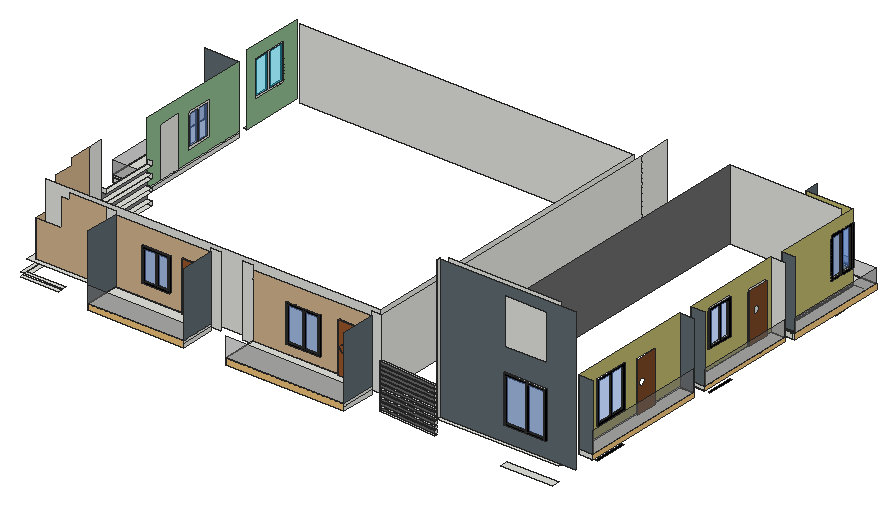
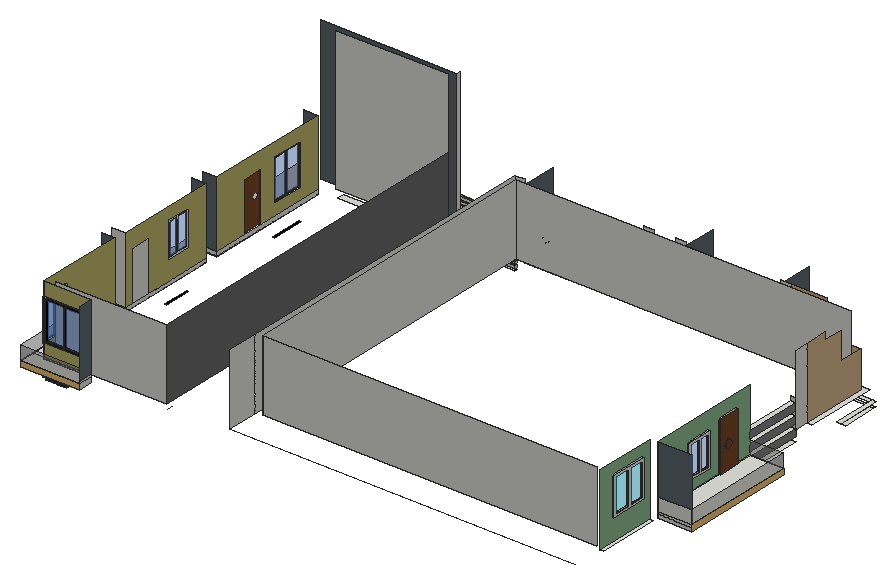
# SketchUp Ruby script. Lengths in inches.
U = 1.inch
M = Sketchup.active_model
def pt(a) = Geom::Point3d.new(a.map { |v| v * U })
def face(e, loops, mat)
  f = e.add_face(loops[0].map { |a| pt(a) })
  loops[1..].each { |l| e.add_face(l.map { |a| pt(a) }).erase! }
  f.material = f.back_material = mat if mat
  f
end
# faces: each face lists its corners as indices into pts; further lists are holes
def faces(e, pts, list, mat = nil) = list.each { |f| face(e, (f[0].is_a?(Array) ? f : [f]).map { |l| l.map { |i| pts[i] } }, mat) }
# xy, xz, yz: faces in a plane at the given z, y or x. An outline is a flat list of corners, or four numbers for a rectangle; further outlines are holes
def ring(l) = l.size == 4 ? [[l[0], l[1]], [l[2], l[1]], [l[2], l[3]], [l[0], l[3]]] : l.each_slice(2).to_a
def flat(e, list, mat, &to3) = list.each { |f| face(e, (f[0].is_a?(Array) ? f : [f]).map { |l| ring(l).map { |u, v| to3.(u, v) } }, mat) }
def xy(e, z, list, mat = nil) = flat(e, list, mat) { |x, y| [x, y, z] }
def xz(e, y, list, mat = nil) = flat(e, list, mat) { |x, z| [x, y, z] }
def yz(e, x, list, mat = nil) = flat(e, list, mat) { |y, z| [x, y, z] }
def lines(e, pts, list) = list.each { |a, b| e.add_line(pt(pts[a]), pt(pts[b])) }
# prism: a flat outline (further loops are holes) pulled along v
def prism(e, loops, v, mat = nil)
  f = face(e, loops, mat); d = Geom::Vector3d.new(v.map { |x| x * U })
  f.pushpull(f.normal.samedirection?(d) ? d.length : -d.length)
end
def box(e, o, s, mat = nil) = prism(e, [[o, [o[0] + s[0], o[1], o[2]], [o[0] + s[0], o[1] + s[1], o[2]], [o[0], o[1] + s[1], o[2]]]], [0, 0, s[2]], mat)
def at(x, y, z, deg = 0) = Geom::Transformation.translation(pt([x, y, z])) * Geom::Transformation.rotation(ORIGIN, Z_AXIS, deg.degrees)
def axes(o, x, y, z) = Geom::Transformation.new([*x, 0, *y, 0, *z, 0, *pt(o).to_a, 1])
def part(name) = M.definitions.add(name)
# library, detail: a bought-in or finely detailed component or shape, given as its bounding box
def library(name, o, s) = part(name).tap { |d| box(d.entities, o, s) }
def detail(e, o, s) = box(e.add_group.entities, o, s)
def put(e, d, t, mat = nil) = e.add_instance(d, t).tap { |i| i.material = mat if mat }
def group(e, t, mat = nil) = e.add_group.tap { |g| g.transformation = t; g.material = mat if mat }.entities
root = M.entities
M.materials.add("[0035_Tan]").color = [210, 180, 140]
M.materials.add("[0057_DarkKhaki]").color = [189, 183, 107]
M.materials.add("[0072_DarkSeaGreen]").color = [143, 188, 143]
M.materials.add("[0133_Gray]").color = [128, 128, 128]
M.materials.add("[0134_DimGray]").color = [105, 105, 105]
M.materials.add("[0137_Black]").color = [0, 0, 0]
M.materials.add("[Formica Speckled Grey]").color = [94, 105, 111]
M.materials.add("[Translucent Glass Blue]").color = [100, 149, 237]
M.materials["[Translucent Glass Blue]"].alpha = 0.5
M.materials.add("[Translucent Glass Gray]").color = [128, 128, 128]
M.materials["[Translucent Glass Gray]"].alpha = 0.5
M.materials.add("[Translucent Glass Tinted]").color = [8, 201, 241]
M.materials["[Translucent Glass Tinted]"].alpha = 0.48
M.materials.add("[Wood Cherry Original]").color = [152, 86, 42]
M.materials.add("[Wood OSB]").color = [240, 195, 122]
M.materials.add("[Wood Veneer 01]").color = [120, 70, 37]
xy(root,225.63,[[972.47,469.23,975.47,514.23]],"[0137_Black]")
xy(root,225.75,[[68.8125,149.58,74.8125,209.08]])
xy(root,225.8125,[[68.8125,143.58,133.51,149.58]])
xy(root,226.04,[[972.47,735.23,975.47,751.36],[972.47,754.32,975.47,767.48]])
xy(root,226.04,[[934.72,770.48,949.25,773.48],[952.09,770.48,969.47,773.48]],"[0137_Black]")
xy(root,227.05,[[972.47,230.95,975.47,286.51]],"[0137_Black]")
xy(root,227.81,[[766.19,148.96,766.41,152.52,668.06,158.52,667.84,154.96]])
xy(root,227.94,[[884.72,140.58,972.47,152.58]])
xy(root,229.04,[[931.72,770.48,975.47,773.48]],"[0137_Black]")
xy(root,230.48,[[766.19,148.96,667.84,154.96,668.06,158.52,766.41,152.52]])
xy(root,232.22,[[763.41,204.89,766.41,224.45]])
xy(root,233.3125,[[68.8125,143.58,74.8125,219.58],[74.8125,143.58,141.375,149.58]])
xy(root,233.37,[[83.8125,295.24,92.8125,392.06]])
xy(root,234.68,[[766.19,148.96,766.41,152.52,668.06,158.52,667.84,154.96]])
xy(root,235.22,[[763.41,201.89,766.41,227.45]])
xy(root,237.36,[[766.19,148.96,667.84,154.96,668.06,158.52,766.41,152.52]])
xy(root,240.81,[[83.8125,295.24,92.8125,392.06]])
xy(root,241.56,[[766.19,148.96,766.41,152.52,668.06,158.52,667.84,154.96]])
xy(root,244.23,[[766.19,148.96,667.84,154.96,668.06,158.52,766.41,152.52]])
xy(root,245.68,[[450.92,100.8,651.23,158.58]],"[Wood OSB]")
xy(root,246.18,[[217.79,100.8,379.72,158.58],[26.03,392.06,83.8125,587.65]],"[Wood OSB]")
xy(root,246.33,[[975.47,621.6875,975.47,770.48,896.3125,770.48,896.3125,794.48,996.47,794.48,996.47,621.6875]],"[Wood OSB]")
xy(root,248.43,[[766.19,148.96,766.41,152.52,668.06,158.52,667.84,154.96]])
xy(root,251.11,[[766.19,148.96,667.84,154.96,668.06,158.52,766.41,152.52]])
xy(root,252.18,[[74.8125,149.58,200.97,149.58,200.97,158.58,83.8125,158.58,83.8125,271.7,74.8125,271.7],[765.79,152.58,766.41,158.58],[766.41,152.58,972.47,158.58],[77.8125,604.3125,83.8125,709.05]])
xy(root,252.43,[[972.47,194.93,996.47,408.53]],"[Wood OSB]")
xy(root,252.81,[[972.47,431.23,996.47,600.85]],"[Wood OSB]")
xy(root,253.31,[[83.8125,295.24,92.8125,392.06]])
xy(root,255.31,[[766.19,148.96,766.41,152.52,668.06,158.52,667.84,154.96]])
xy(root,255.33,[[975.47,621.6875,996.47,621.6875,996.47,794.48,896.3125,794.48,896.3125,770.48,975.47,770.48]])
xy(root,256.06,[[26.03,392.06,83.8125,392.06,83.8125,421.71,80.8125,421.71,80.8125,457.71,83.8125,457.71,83.8125,587.65,26.03,587.65],[80.8125,421.71,83.8125,457.71]])
xy(root,256.47,[[217.79,100.8,379.72,100.8,379.72,158.58,368.04,158.58,368.04,155.58,332.04,155.58,332.04,158.58,217.79,158.58],[332.04,155.58,368.04,158.58]])
xy(root,256.72,[[450.92,100.8,651.23,100.8,651.23,158.58,632.81,158.58,632.81,155.58,596.81,155.58,596.81,158.58,450.92,158.58],[596.81,155.58,632.81,158.58]])
xy(root,257.98,[[766.19,148.96,667.84,154.96,668.06,158.52,766.41,152.52]])
xy(root,259.18,[[972.47,431.23,996.47,431.23,996.47,600.85,972.47,600.85,972.47,589.32,975.47,589.32,975.47,553.32,972.47,553.32],[972.47,553.32,975.47,589.32]])
xy(root,259.44,[[972.47,194.93,996.47,194.93,996.47,408.53,972.47,408.53,972.47,351.42,975.47,351.42,975.47,315.42,972.47,315.42],[972.47,315.42,975.47,351.42]])
xy(root,260.75,[[83.8125,295.24,92.8125,392.06]])
xy(root,262.18,[[766.19,148.96,766.41,152.52,668.06,158.52,667.84,154.96]])
xy(root,264.86,[[766.19,148.96,667.84,154.96,668.06,158.52,766.41,152.52]])
xy(root,269.06,[[766.19,148.96,766.41,152.52,668.06,158.52,667.84,154.96]])
xy(root,271.73,[[766.19,148.96,667.84,154.96,668.06,158.52,766.41,152.52]])
xy(root,273.11,[[508.66,155.58,565.66,158.58]])
xy(root,273.25,[[83.8125,295.24,92.8125,392.06]])
xy(root,275.6,[[80.8125,480.71,83.8125,524.33]])
xy(root,275.93,[[766.19,148.96,766.41,152.52,668.06,158.52,667.84,154.96]])
xy(root,276.11,[[511.66,155.58,537.16,158.58],[540.07,155.58,562.66,158.58]],"[0137_Black]")
xy(root,278.6,[[80.8125,483.71,83.8125,500.7],[80.8125,502.52,83.8125,521.33]])
xy(root,278.61,[[766.19,148.96,667.84,154.96,668.06,158.52,766.41,152.52]])
xy(root,278.71,[[972.47,231.45,975.47,288.58]])
xy(root,279.84,[[877.02,155.58,947.52,158.58]],"[0137_Black]")
xy(root,280.21,[[264.42,155.58,311.74,158.58]])
xy(root,280.69,[[83.8125,295.24,92.8125,392.06]])
xy(root,281.03,[[972.47,725.48,975.47,770.48],[903.22,770.48,972.47,773.48],[972.47,770.48,975.47,773.48]])
xy(root,281.71,[[972.47,234.45,975.47,260.01],[972.47,262.22,975.47,285.58]],"[0137_Black]")
xy(root,282.81,[[766.19,148.96,766.41,152.52,668.06,158.52,667.84,154.96]])
xy(root,282.84,[[914.48,155.58,916.69,158.58]])
xy(root,282.84,[[880.02,155.58,912.27,158.58],[912.27,155.58,914.48,158.58],[916.69,155.58,944.52,158.58]],"[0137_Black]")
xy(root,283.21,[[267.42,155.58,288.08,158.58],[291.62,155.58,308.74,158.58]],"[0137_Black]")
xy(root,284.03,[[972.47,728.48,975.47,747.98],[972.47,750.32,975.47,767.48],[906.22,770.48,937.84,773.48],[940.13,770.48,969.47,773.48]],"[0137_Black]")
xy(root,285.48,[[766.19,148.96,667.84,154.96,668.06,158.52,766.41,152.52]])
xy(root,289.68,[[766.19,148.96,766.41,152.52,668.06,158.52,667.84,154.96]])
xy(root,290.04,[[80.8125,620.08,83.8125,683.08]])
xy(root,291.73,[[972.47,468.54,975.47,512.23]])
xy(root,292.36,[[766.19,148.96,667.84,154.96,668.06,158.52,766.41,152.52]])
xy(root,293.04,[[80.8125,623.08,83.8125,648.35],[80.8125,651.58,83.8125,680.08]])
xy(root,293.18,[[83.8125,295.24,92.8125,392.06]])
xy(root,294.73,[[972.47,471.54,975.47,490.38],[972.47,492.52,975.47,509.23]],"[0137_Black]")
xy(root,296.56,[[766.19,148.96,766.41,152.52,668.06,158.52,667.84,154.96]])
xy(root,299.23,[[766.19,148.96,667.84,154.96,668.06,158.52,766.41,152.52]])
xz(root,100.8,[[217.79,256.47,379.72,284.7],[450.92,256.72,651.23,288.66]],"[Translucent Glass Gray]")
xz(root,100.8,[[450.92,245.68,651.23,256.72],[217.79,246.18,379.72,256.47]],"[Wood OSB]")
xz(root,152.58,[[765.79,252.18,766.41,492.18]])
xz(root,152.58,[[345.48,293.71,347.13,293.92,348.67,294.56,349.99,295.57,351,296.89,351.64,298.43,351.85,300.08,351.64,301.73,351,303.27,349.99,304.59,348.67,305.6,347.13,306.24,345.48,306.46,343.83,306.24,342.29,305.6,340.97,304.59,339.96,303.27,339.32,301.73,339.1,300.08,339.32,298.43,339.96,296.89,340.97,295.57,342.29,294.56,343.83,293.92],[608.1,295.62,609.59,295.8125,610.97,296.39,612.16,297.3,613.08,298.49,613.65,299.88,613.85,301.37,613.65,302.85,613.08,304.24,612.16,305.43,610.97,306.35,609.59,306.92,608.1,307.12,606.61,306.92,605.22,306.35,604.03,305.43,603.12,304.24,602.54,302.85,602.35,301.37,602.54,299.88,603.12,298.49,604.03,297.3,605.22,296.39,606.61,295.8125]],"[Wood Cherry Original]")
xz(root,155.58,[[608.1,295.62,606.61,295.8125,605.22,296.39,604.03,297.3,603.12,298.49,602.54,299.88,602.35,301.37,602.54,302.85,603.12,304.24,604.03,305.43,605.22,306.35,606.61,306.92,608.1,307.12,609.59,306.92,610.97,306.35,612.16,305.43,613.08,304.24,613.65,302.85,613.85,301.37,613.65,299.88,613.08,298.49,612.16,297.3,610.97,296.39,609.59,295.8125]])
xz(root,155.58,[[[508.66,273.11,565.66,336.43],[511.66,276.11,537.16,333.43],[540.07,276.11,562.66,333.43]],[[877.02,279.84,947.52,358.59],[880.02,282.84,944.52,355.59]],[[264.42,280.21,311.74,336.34],[267.42,283.21,288.08,333.34],[291.62,283.21,308.74,333.34]],[914.48,282.84,916.69,355.59]],"[0137_Black]")
xz(root,155.58,[[[332.04,256.47,368.04,340.47],[345.48,293.71,343.83,293.92,342.29,294.56,340.97,295.57,339.96,296.89,339.32,298.43,339.1,300.08,339.32,301.73,339.96,303.27,340.97,304.59,342.29,305.6,343.83,306.24,345.48,306.46,347.13,306.24,348.67,305.6,349.99,304.59,351,303.27,351.64,301.73,351.85,300.08,351.64,298.43,351,296.89,349.99,295.57,348.67,294.56,347.13,293.92]],[[596.81,256.72,632.81,340.72],[608.1,295.62,606.61,295.8125,605.22,296.39,604.03,297.3,603.12,298.49,602.54,299.88,602.35,301.37,602.54,302.85,603.12,304.24,604.03,305.43,605.22,306.35,606.61,306.92,608.1,307.12,609.59,306.92,610.97,306.35,612.16,305.43,613.08,304.24,613.65,302.85,613.85,301.37,613.65,299.88,613.08,298.49,612.16,297.3,610.97,296.39,609.59,295.8125]]],"[Wood Cherry Original]")
xz(root,158.58,[[450.92,245.68,651.23,252.18],[217.79,246.18,379.72,252.18],[200.97,252.18,217.79,372.18],[217.79,252.18,379.72,256.47],[379.72,252.18,396.54,372.18],
  [434.03,252.18,450.85,372.18],[450.92,252.18,651.23,256.72],[651.23,252.18,668.06,372.18],[765.79,252.18,766.41,372.18],[332.04,256.47,368.04,340.47],
  [596.81,256.72,632.81,340.72],[[508.66,273.11,565.66,336.43],[511.66,276.11,537.16,333.43],[540.07,276.11,562.66,333.43]],[[877.02,279.84,947.52,358.59],[880.02,282.84,944.52,355.59]],[[264.42,280.21,311.74,336.34],[267.42,283.21,288.08,333.34],[291.62,283.21,308.74,333.34]],[914.48,282.84,916.69,355.59]])
xz(root,158.58,[[83.8125,252.18,200.97,252.18,200.97,372.18,141.375,372.18,141.375,360.74,126.6875,360.74,126.6875,314.18,83.8125,314.18],[[450.85,252.18,450.92,252.18,450.92,256.72,596.81,256.72,596.81,340.72,632.81,340.72,632.81,256.72,651.23,256.72,651.23,364.37,450.92,364.37,450.92,372.18,450.85,372.18],[508.66,273.11,565.66,336.43]],[[217.79,256.47,332.04,256.47,332.04,340.47,368.04,340.47,368.04,256.47,379.72,256.47,379.72,366.18,217.79,366.18],[264.42,280.21,311.74,336.34]]],"[0035_Tan]")
xz(root,158.58,[[[766.41,252.18,996.47,492.18],[877.02,279.84,947.52,358.59],[877.02,396.78,947.52,475.53]]],"[Formica Speckled Grey]")
xz(root,158.58,[[511.66,276.11,537.16,333.43],[540.07,276.11,562.66,333.43],[880.02,282.84,914.48,355.59],[916.69,282.84,944.52,355.59],[267.42,283.21,288.08,333.34],
  [291.62,283.21,308.74,333.34]],"[Translucent Glass Blue]")
xz(root,167.52,[[608.1,295.62,606.61,295.8125,605.22,296.39,604.03,297.3,603.12,298.49,602.54,299.88,602.35,301.37,602.54,302.85,603.12,304.24,604.03,305.43,605.22,306.35,606.61,306.92,608.1,307.12,609.59,306.92,610.97,306.35,612.16,305.43,613.08,304.24,613.65,302.85,613.85,301.37,613.65,299.88,613.08,298.49,612.16,297.3,610.97,296.39,609.59,295.8125]])
xz(root,167.58,[[92.8125,252.18,659.06,372.18],[775.41,252.18,963.47,492.18]])
xz(root,194.93,[[972.47,252.18,996.47,252.43],[972.47,252.43,996.47,259.44]])
xz(root,194.93,[[972.47,259.44,996.47,372.18]],"[Formica Speckled Grey]")
xz(root,231.45,[[972.47,278.71,975.47,349.83]],"[0137_Black]")
xz(root,234.45,[[972.47,281.71,975.47,346.83]],"[0137_Black]")
xz(root,260.01,[[972.47,281.71,975.47,346.83]],"[0137_Black]")
xz(root,262.22,[[972.47,281.71,975.47,346.83]],"[0137_Black]")
xz(root,285.58,[[972.47,281.71,975.47,346.83]],"[0137_Black]")
xz(root,288.58,[[972.47,278.71,975.47,349.83]],"[0137_Black]")
xz(root,295.24,[[83.8125,253.31,92.8125,260.75],[83.8125,273.25,92.8125,280.69],[83.8125,293.18,92.8125,300.63]])
xz(root,315.42,[[972.47,259.44,975.47,343.44]],"[Wood Veneer 01]")
xz(root,351.42,[[972.47,259.44,975.47,343.44]],"[Wood Veneer 01]")
xz(root,392.06,[[83.8125,233.37,92.8125,240.81],[26.03,246.18,83.8125,252.18],[26.03,252.18,83.8125,252.56],[26.03,252.56,83.8125,253.31],[26.03,253.31,83.8125,256.06],
  [83.8125,253.31,92.8125,260.75],[83.8125,273.25,92.8125,280.69],[83.8125,293.18,92.8125,300.63]])
xz(root,392.06,[[26.03,256.06,83.8125,279.26]],"[Translucent Glass Gray]")
xz(root,408.53,[[972.47,252.18,996.47,252.43],[972.47,252.43,996.47,259.44]])
xz(root,408.53,[[972.47,259.44,996.47,372.18]],"[Formica Speckled Grey]")
xz(root,421.71,[[80.8125,256.06,83.8125,340.06]],"[Wood Veneer 01]")
xz(root,431.23,[[972.47,252.18,996.47,252.81],[972.47,252.81,996.47,259.18]])
xz(root,431.23,[[972.47,259.18,996.47,372.18]],"[Formica Speckled Grey]")
xz(root,457.71,[[80.8125,256.06,83.8125,340.06]],"[Wood Veneer 01]")
xz(root,468.54,[[972.47,291.73,975.47,352.41]],"[0137_Black]")
xz(root,471.54,[[972.47,294.73,975.47,349.41]],"[0137_Black]")
xz(root,480.71,[[80.8125,275.6,83.8125,332.54]])
xz(root,483.71,[[80.8125,278.6,83.8125,329.54]])
xz(root,490.38,[[972.47,294.73,975.47,349.41]],"[0137_Black]")
xz(root,492.52,[[972.47,294.73,975.47,349.41]],"[0137_Black]")
xz(root,500.7,[[80.8125,278.6,83.8125,329.54]])
xz(root,502.52,[[80.8125,278.6,83.8125,329.54]])
xz(root,509.23,[[972.47,294.73,975.47,349.41]],"[0137_Black]")
xz(root,512.23,[[972.47,291.73,975.47,352.41]],"[0137_Black]")
xz(root,521.33,[[80.8125,278.6,83.8125,329.54]])
xz(root,524.33,[[80.8125,275.6,83.8125,332.54]])
xz(root,553.32,[[972.47,259.18,975.47,343.18]],"[Wood Veneer 01]")
xz(root,587.65,[[26.03,246.18,83.8125,252.18],[26.03,252.18,83.8125,256.06],[26.03,256.06,83.8125,279.26]])
xz(root,587.65,[[26.03,279.26,83.8125,362.62]],"[Formica Speckled Grey]")
xz(root,589.32,[[972.47,259.18,975.47,343.18]],"[Wood Veneer 01]")
xz(root,600.85,[[972.47,252.18,996.47,252.81],[972.47,252.81,996.47,259.18],[972.47,259.18,996.47,372.18]])
xz(root,620.08,[[80.8125,290.04,83.8125,353.04]])
xz(root,621.6875,[[975.47,246.33,993.47,255.33],[993.47,246.33,996.47,255.33],[975.47,255.33,993.47,255.4],[993.47,255.33,996.47,255.4],[975.47,255.4,993.47,257.58],
  [993.47,255.4,996.47,257.58],[975.47,257.58,993.47,258.33],[993.47,257.58,996.47,258.33]])
xz(root,621.6875,[[975.47,258.33,996.47,372.33]],"[Formica Speckled Grey]")
xz(root,623.08,[[80.8125,293.04,83.8125,350.04]])
xz(root,648.35,[[80.8125,293.04,83.8125,350.04]])
xz(root,651.58,[[80.8125,293.04,83.8125,350.04]])
xz(root,680.08,[[80.8125,293.04,83.8125,350.04]])
xz(root,683.08,[[80.8125,290.04,83.8125,353.04]])
xz(root,703.7,[[92.8125,252.18,659.06,372.18]])
xz(root,725.48,[[972.47,281.03,975.47,350.28]])
xz(root,728.48,[[972.47,284.03,975.47,347.28]],"[0137_Black]")
xz(root,747.98,[[972.47,284.03,975.47,347.28]])
xz(root,750.32,[[972.47,284.03,975.47,347.28]],"[0137_Black]")
xz(root,761.48,[[775.41,252.18,963.47,372.18]])
xz(root,767.48,[[972.47,284.03,975.47,347.28]])
xz(root,770.48,[[896.3125,246.33,918.4,255.33],[918.4,246.33,975.47,255.33],[896.3125,255.33,918.4,258.33],[918.4,255.33,975.47,258.33],[[903.22,281.03,972.47,350.28],[906.22,284.03,937.84,347.28],[940.13,284.03,969.47,347.28]],
  [972.47,281.03,975.47,350.28]])
xz(root,770.48,[[896.3125,258.33,896.3125,372.33,975.47,372.33,975.47,350.28,903.22,350.28,903.22,281.03,975.47,281.03,975.47,258.33]],"[0057_DarkKhaki]")
xz(root,770.48,[[906.22,284.03,937.84,347.28],[940.13,284.03,969.47,347.28]],"[Translucent Glass Blue]")
xz(root,773.48,[[[903.22,281.03,972.47,350.28],[906.22,284.03,937.84,347.28],[940.13,284.03,969.47,347.28]],[972.47,281.03,975.47,350.28]],"[0137_Black]")
xz(root,794.48,[[896.3125,255.33,996.47,278.97]],"[Translucent Glass Gray]")
xz(root,794.48,[[896.3125,246.33,996.47,255.33]],"[Wood OSB]")
yz(root,26.03,[[392.06,256.06,587.65,279.26]],"[Translucent Glass Gray]")
yz(root,26.03,[[392.06,246.18,587.65,256.06]],"[Wood OSB]")
yz(root,77.8125,[[443.41,292.11,441.92,292.31,440.54,292.88,439.35,293.79,438.43,294.98,437.86,296.37,437.66,297.86,437.86,299.35,438.43,300.73,439.35,301.93,440.54,302.84,441.92,303.41,443.41,303.61,444.9,303.41,446.29,302.84,447.48,301.93,448.39,300.73,448.97,299.35,449.16,297.86,448.97,296.37,448.39,294.98,447.48,293.79,446.29,292.88,444.9,292.31]],"[Wood Veneer 01]")
yz(root,80.8125,[[[480.71,275.6,524.33,332.54],[502.52,278.6,521.33,329.54],[483.71,278.6,500.7,329.54]],[[620.08,290.04,683.08,353.04],[651.58,293.04,680.08,350.04],[623.08,293.04,648.35,350.04]],[443.41,292.11,444.9,292.31,446.29,292.88,447.48,293.79,448.39,294.98,448.97,296.37,449.16,297.86,448.97,299.35,448.39,300.73,447.48,301.93,446.29,302.84,444.9,303.41,443.41,303.61,441.92,303.41,440.54,302.84,439.35,301.93,438.43,300.73,437.86,299.35,437.66,297.86,437.86,296.37,438.43,294.98,439.35,293.79,440.54,292.88,441.92,292.31]])
yz(root,80.8125,[[[421.71,256.06,457.71,340.06],[443.41,292.11,444.9,292.31,446.29,292.88,447.48,293.79,448.39,294.98,448.97,296.37,449.16,297.86,448.97,299.35,448.39,300.73,447.48,301.93,446.29,302.84,444.9,303.41,443.41,303.61,441.92,303.41,440.54,302.84,439.35,301.93,438.43,300.73,437.86,299.35,437.66,297.86,437.86,296.37,438.43,294.98,439.35,293.79,440.54,292.88,441.92,292.31]]],"[Wood Veneer 01]")
yz(root,83.8125,[[392.06,246.18,587.65,252.18],[271.7,252.18,295.24,372.18],[392.06,252.18,587.65,256.06],[421.71,256.06,457.71,340.06],[[480.71,275.6,524.33,332.54],[502.52,278.6,521.33,329.54],[483.71,278.6,500.7,329.54]],
  [[620.08,290.04,683.08,353.04],[651.58,293.04,680.08,350.04],[623.08,293.04,648.35,350.04]]])
yz(root,83.8125,[[158.58,252.18,158.58,314.24,200.33,314.24,200.33,360.74,232.98,360.74,232.98,372.18,271.7,372.18,271.7,252.18]],"[0035_Tan]")
yz(root,83.8125,[[[604.3125,252.18,709.05,372.18],[620.08,290.04,683.08,353.04]],[[392.06,256.06,392.06,362.62,587.65,362.62,587.65,256.06,457.71,256.06,457.71,340.06,421.71,340.06,421.71,256.06],[480.71,275.6,524.33,332.54]]],"[0072_DarkSeaGreen]")
yz(root,83.8125,[[295.24,240.81,392.06,253.31],[295.24,260.75,392.06,273.25],[295.24,280.69,392.06,293.18]],"[0133_Gray]")
yz(root,83.8125,[[483.71,278.6,500.7,329.54],[502.52,278.6,521.33,329.54]],"[Translucent Glass Blue]")
yz(root,83.8125,[[623.08,293.04,648.35,350.04],[651.58,293.04,680.08,350.04]],"[Translucent Glass Tinted]")
yz(root,217.79,[[100.8,246.18,158.58,252.18],[100.8,252.18,158.58,256.47]])
yz(root,217.79,[[100.8,256.47,158.58,366.18]],"[Formica Speckled Grey]")
yz(root,264.42,[[155.58,280.21,158.58,336.34]],"[0137_Black]")
yz(root,267.42,[[155.58,283.21,158.58,333.34]],"[0137_Black]")
yz(root,288.08,[[155.58,283.21,158.58,333.34]],"[0137_Black]")
yz(root,291.62,[[155.58,283.21,158.58,333.34]],"[0137_Black]")
yz(root,308.74,[[155.58,283.21,158.58,333.34]],"[0137_Black]")
yz(root,311.74,[[155.58,280.21,158.58,336.34]],"[0137_Black]")
yz(root,332.04,[[155.58,256.47,158.58,340.47]],"[Wood Cherry Original]")
yz(root,368.04,[[155.58,256.47,158.58,340.47]],"[Wood Cherry Original]")
yz(root,379.72,[[100.8,246.18,158.58,252.18],[100.8,252.18,158.58,256.47]])
yz(root,379.72,[[100.8,256.47,158.58,366.18]],"[Formica Speckled Grey]")
yz(root,450.92,[[100.8,245.68,158.58,252.18],[100.8,252.18,158.58,256.72]])
yz(root,508.66,[[155.58,273.11,158.58,336.43]],"[0137_Black]")
yz(root,511.66,[[155.58,276.11,158.58,333.43]],"[0137_Black]")
yz(root,537.16,[[155.58,276.11,158.58,333.43]],"[0137_Black]")
yz(root,540.07,[[155.58,276.11,158.58,333.43]],"[0137_Black]")
yz(root,562.66,[[155.58,276.11,158.58,333.43]],"[0137_Black]")
yz(root,565.66,[[155.58,273.11,158.58,336.43]],"[0137_Black]")
yz(root,596.81,[[155.58,256.72,158.58,340.72]],"[Wood Cherry Original]")
yz(root,632.81,[[155.58,256.72,158.58,340.72]],"[Wood Cherry Original]")
yz(root,651.23,[[100.8,245.68,158.58,252.18],[100.8,252.18,158.58,256.72]])
yz(root,651.23,[[100.8,256.72,158.58,364.37]],"[Formica Speckled Grey]")
yz(root,659.06,[[167.58,252.18,703.7,372.18]])
yz(root,668.06,[[158.58,252.18,709.05,372.18],[709.05,252.18,761.48,372.18]])
yz(root,765.79,[[152.58,252.18,158.58,492.18]])
yz(root,766.41,[[152.52,252.18,152.58,492.18],[152.58,252.18,158.58,492.18]])
yz(root,775.41,[[167.58,252.18,761.48,372.18]],"[0134_DimGray]")
yz(root,877.02,[[155.58,279.84,158.58,358.59]],"[0137_Black]")
yz(root,880.02,[[155.58,282.84,158.58,355.59]],"[0137_Black]")
yz(root,896.3125,[[770.48,246.33,794.48,255.33],[770.48,255.33,794.48,258.33]])
yz(root,896.3125,[[770.48,258.33,794.48,372.33]],"[Formica Speckled Grey]")
yz(root,903.22,[[770.48,281.03,773.48,350.28]],"[0137_Black]")
yz(root,906.22,[[770.48,284.03,773.48,347.28]],"[0137_Black]")
yz(root,914.48,[[155.58,282.84,158.58,355.59]],"[0137_Black]")
yz(root,916.69,[[155.58,282.84,158.58,355.59]],"[0137_Black]")
yz(root,937.84,[[770.48,284.03,773.48,347.28]],"[0137_Black]")
yz(root,940.13,[[770.48,284.03,773.48,347.28]],"[0137_Black]")
yz(root,944.52,[[155.58,282.84,158.58,355.59]],"[0137_Black]")
yz(root,947.52,[[155.58,279.84,158.58,358.59]],"[0137_Black]")
yz(root,969.47,[[770.48,284.03,773.48,347.28]],"[0137_Black]")
yz(root,972.47,[[194.93,252.18,408.53,252.43],[431.23,252.18,600.85,252.81],[194.93,252.43,408.53,259.44],[431.23,252.81,600.85,259.18],[553.32,259.18,589.32,343.18],
  [[725.48,281.03,770.48,350.28],[728.48,284.03,747.98,347.28],[750.32,284.03,767.48,347.28]],[770.48,281.03,773.48,350.28],[[468.54,291.73,512.23,352.41],[471.54,294.73,490.38,349.41],[492.52,294.73,509.23,349.41]]])
yz(root,972.47,[[[431.23,259.18,553.32,259.18,553.32,343.18,589.32,343.18,589.32,259.18,600.85,259.18,600.85,372.18,431.23,372.18],[468.54,291.73,512.23,352.41]],[[194.93,259.44,315.42,259.44,315.42,343.44,351.42,343.44,351.42,259.44,408.53,259.44,408.53,372.18,194.93,372.18],[231.45,278.71,288.58,349.83]]],"[0057_DarkKhaki]")
yz(root,972.47,[[234.45,281.71,260.01,346.83],[262.22,281.71,285.58,346.83],[728.48,284.03,747.98,347.28],[750.32,284.03,767.48,347.28],[471.54,294.73,490.38,349.41],
  [492.52,294.73,509.23,349.41]],"[Translucent Glass Blue]")
yz(root,975.47,[[621.6875,246.33,770.48,255.33],[621.6875,255.33,770.48,255.4],[621.6875,255.4,770.48,257.58],[621.6875,257.58,770.48,258.33]])
yz(root,975.47,[[621.6875,258.33,770.48,258.33,770.48,281.03,725.48,281.03,725.48,350.28,770.48,350.28,770.48,372.33,621.6875,372.33]],"[0057_DarkKhaki]")
yz(root,975.47,[[[231.45,278.71,288.58,349.83],[234.45,281.71,260.01,346.83],[262.22,281.71,285.58,346.83]],[[725.48,281.03,770.48,350.28],[728.48,284.03,747.98,347.28],[750.32,284.03,767.48,347.28]],[770.48,281.03,773.48,350.28],[[468.54,291.73,512.23,352.41],[471.54,294.73,490.38,349.41],[492.52,294.73,509.23,349.41]]],"[0137_Black]")
yz(root,975.47,[[[553.32,259.18,589.32,343.18],[566.66,302.99,565.11,303.19,563.66,303.79,562.42,304.75,561.46,305.99,560.86,307.4375,560.66,308.99,560.86,310.54,561.46,311.99,562.42,313.23,563.66,314.19,565.11,314.78,566.66,314.99,568.21,314.78,569.66,314.19,570.9,313.23,571.86,311.99,572.46,310.54,572.66,308.99,572.46,307.4375,571.86,305.99,570.9,304.75,569.66,303.79,568.21,303.19]],[[315.42,259.44,351.42,343.44],[324.66,300.15,323.16,300.35,321.76,300.93,320.55,301.85,319.63,303.05,319.05,304.46,318.85,305.96,319.05,307.46,319.63,308.87,320.55,310.07,321.76,310.99,323.16,311.57,324.66,311.77,326.17,311.57,327.57,310.99,328.77,310.07,329.7,308.87,330.28,307.46,330.47,305.96,330.28,304.46,329.7,303.05,328.77,301.85,327.57,300.93,326.17,300.35]]],"[Wood Veneer 01]")
yz(root,996.47,[[621.6875,255.33,794.48,278.97],[431.23,259.18,600.85,285.2],[194.93,259.44,408.53,295.67]],"[Translucent Glass Gray]")
yz(root,996.47,[[621.6875,246.33,794.48,255.33],[194.93,252.43,408.53,259.44],[431.23,252.81,600.85,259.18]],"[Wood OSB]")
p = [[766.19,148.96,234.68],[667.84,154.96,234.68],[667.84,154.96,230.48],[766.19,148.96,230.48],[766.41,152.52,230.48],[766.41,152.52,234.68],
  [668.06,158.52,234.68],[668.06,158.52,230.48],[766.19,148.96,241.56],[667.84,154.96,241.56],[667.84,154.96,237.36],[766.19,148.96,237.36],
  [766.41,152.52,237.36],[766.41,152.52,241.56],[668.06,158.52,241.56],[668.06,158.52,237.36],[766.19,148.96,248.43],[667.84,154.96,248.43],
  [667.84,154.96,244.23],[766.19,148.96,244.23],[766.41,152.52,244.23],[766.41,152.52,248.43],[668.06,158.52,248.43],[668.06,158.52,244.23],
  [766.19,148.96,255.31],[667.84,154.96,255.31],[667.84,154.96,251.11],[766.19,148.96,251.11],[766.19,148.96,252.18],[766.41,152.52,251.11],
  [766.41,152.52,252.18],[668.06,158.52,255.31],[766.41,152.52,255.31],[668.06,158.52,251.11],[668.06,158.58,372.18],[668.06,158.58,252.18],
  [668.05,158.52,252.18],[668.05,158.52,372.18],[766.19,148.96,262.18],[667.84,154.96,262.18],[667.84,154.96,257.98],[766.19,148.96,257.98],
  [766.41,152.52,257.98],[766.41,152.52,262.18],[668.06,158.52,262.18],[668.06,158.52,257.98],[766.19,148.96,269.06],[667.84,154.96,269.06],
  [667.84,154.96,264.86],[766.19,148.96,264.86],[766.41,152.52,264.86],[766.41,152.52,269.06],[668.06,158.52,269.06],[668.06,158.52,264.86],
  [766.19,148.96,275.93],[667.84,154.96,275.93],[667.84,154.96,271.73],[766.19,148.96,271.73],[766.41,152.52,271.73],[766.41,152.52,275.93],
  [668.06,158.52,275.93],[668.06,158.52,271.73],[766.19,148.96,282.81],[667.84,154.96,282.81],[667.84,154.96,278.61],[766.19,148.96,278.61],
  [766.41,152.52,278.61],[766.41,152.52,282.81],[668.06,158.52,282.81],[668.06,158.52,278.61],[766.19,148.96,289.68],[667.84,154.96,289.68],
  [667.84,154.96,285.48],[766.19,148.96,285.48],[766.41,152.52,285.48],[766.41,152.52,289.68],[668.06,158.52,289.68],[668.06,158.52,285.48],
  [80.8125,443.41,292.11],[80.8125,441.92,292.31],[77.8125,441.92,292.31],[77.8125,443.41,292.11],[80.8125,444.9,292.31],[77.8125,444.9,292.31],
  [80.8125,440.54,292.88],[77.8125,440.54,292.88],[80.8125,446.29,292.88],[77.8125,446.29,292.88],[766.19,148.96,296.56],[667.84,154.96,296.56],
  [667.84,154.96,292.36],[766.19,148.96,292.36],[766.41,152.52,292.36],[766.41,152.52,296.56],[668.06,158.52,296.56],[668.06,158.52,292.36],
  [80.8125,439.35,293.79],[77.8125,439.35,293.79],[80.8125,447.48,293.79],[77.8125,447.48,293.79],[343.83,155.58,293.92],[345.48,155.58,293.71],
  [345.48,152.58,293.71],[343.83,152.58,293.92],[347.13,155.58,293.92],[347.13,152.58,293.92],[80.8125,438.43,294.98],[77.8125,438.43,294.98],
  [80.8125,448.39,294.98],[77.8125,448.39,294.98],[342.29,155.58,294.56],[342.29,152.58,294.56],[348.67,155.58,294.56],[348.67,152.58,294.56],
  [340.97,155.58,295.57],[340.97,152.58,295.57],[349.99,155.58,295.57],[349.99,152.58,295.57],[80.8125,437.86,296.37],[77.8125,437.86,296.37],
  [80.8125,448.97,296.37],[77.8125,448.97,296.37],[339.96,155.58,296.89],[339.96,152.58,296.89],[351,155.58,296.89],[351,152.58,296.89],
  [606.61,155.58,295.8125],[608.1,155.58,295.62],[608.1,152.58,295.62],[606.61,152.58,295.8125],[609.59,155.58,295.8125],[609.59,152.58,295.8125],
  [606.61,167.52,295.8125],[608.1,167.52,295.62],[609.59,167.52,295.8125],[605.22,155.58,296.39],[605.22,152.58,296.39],[610.97,155.58,296.39],
  [610.97,152.58,296.39],[605.22,167.52,296.39],[610.97,167.52,296.39],[604.03,155.58,297.3],[604.03,152.58,297.3],[612.16,155.58,297.3],
  [612.16,152.58,297.3],[604.03,167.52,297.3],[612.16,167.52,297.3],[80.8125,437.66,297.86],[77.8125,437.66,297.86],[80.8125,449.16,297.86],
  [77.8125,449.16,297.86],[339.32,155.58,298.43],[339.32,152.58,298.43],[351.64,155.58,298.43],[351.64,152.58,298.43],[603.12,155.58,298.49],
  [603.12,152.58,298.49],[613.08,155.58,298.49],[613.08,152.58,298.49],[603.12,167.52,298.49],[613.08,167.52,298.49],[80.8125,437.86,299.35],
  [77.8125,437.86,299.35],[80.8125,448.97,299.35],[77.8125,448.97,299.35],[339.1,155.58,300.08],[339.1,152.58,300.08],[351.85,155.58,300.08],
  [351.85,152.58,300.08],[602.54,155.58,299.88],[602.54,152.58,299.88],[613.65,155.58,299.88],[613.65,152.58,299.88],[602.54,167.52,299.88],
  [613.65,167.52,299.88],[766.19,148.96,303.43],[667.84,154.96,303.43],[667.84,154.96,299.23],[766.19,148.96,299.23],[766.41,152.52,299.23],
  [766.41,152.52,303.43],[668.06,158.52,303.43],[668.06,158.52,299.23],[80.8125,438.43,300.73],[77.8125,438.43,300.73],[80.8125,448.39,300.73],
  [77.8125,448.39,300.73],[766.41,761.48,252.18],[766.41,770.48,252.18],[668.06,761.48,252.18],[83.8125,761.48,252.18],[975.47,770.48,257.58],
  [993.47,770.48,257.58],[993.47,770.48,255.4],[993.47,770.48,255.33]]
faces(root,p,[[0,1,2,3],[8,9,10,11],[16,17,18,19],[24,25,26,27,28],[38,39,40,41],[46,47,48,49],[54,55,56,57],[62,63,64,65],
  [70,71,72,73],[88,89,90,91],[175,176,177,178]],"[0134_DimGray]")
faces(root,p,[[4,5,0,3],[6,5,4,7],[6,7,2,1],[12,13,8,11],[14,13,12,15],[14,15,10,9],[20,21,16,19],[22,21,20,23],
  [22,23,18,17],[29,30,28,27],[31,32,30,29,33],[31,33,26,25],[30,32,24,28],[34,35,36,37],[42,43,38,41],[44,43,42,45],
  [44,45,40,39],[50,51,46,49],[52,51,50,53],[52,53,48,47],[58,59,54,57],[60,59,58,61],[60,61,56,55],[66,67,62,65],
  [68,67,66,69],[68,69,64,63],[74,75,70,73],[76,75,74,77],[76,77,72,71],[92,93,88,91],[94,93,92,95],[94,95,90,89],
  [127,126,132,133],[130,127,133,134],[126,135,139,132],[137,130,134,140],[135,141,145,139],[143,137,140,146],[141,155,159,145],[157,143,146,160],
  [155,169,173,159],[171,157,160,174],[179,180,175,178],[181,180,179,182],[181,182,177,176]])
faces(root,p,[[78,79,80,81],[82,78,81,83],[79,84,85,80],[86,82,83,87],[84,96,97,85],[98,86,87,99],[96,106,107,97],[108,98,99,109],
  [106,118,119,107],[120,108,109,121],[118,147,148,119],[149,120,121,150],[147,161,162,148],[163,149,150,164],[161,183,184,162],[185,163,164,186]],"[Wood Veneer 01]")
faces(root,p,[[100,101,102,103],[101,104,105,102],[110,100,103,111],[104,112,113,105],[114,110,111,115],[112,116,117,113],[122,114,115,123],[116,124,125,117],
  [126,127,128,129],[127,130,131,128],[135,126,129,136],[130,137,138,131],[141,135,136,142],[137,143,144,138],[151,122,123,152],[124,153,154,125],
  [155,141,142,156],[143,157,158,144],[165,151,152,166],[153,167,168,154],[169,155,156,170],[157,171,172,158]],"[Wood Cherry Original]")
lines(root,p,[[187,188],[189,190],[191,192],[193,194]])
